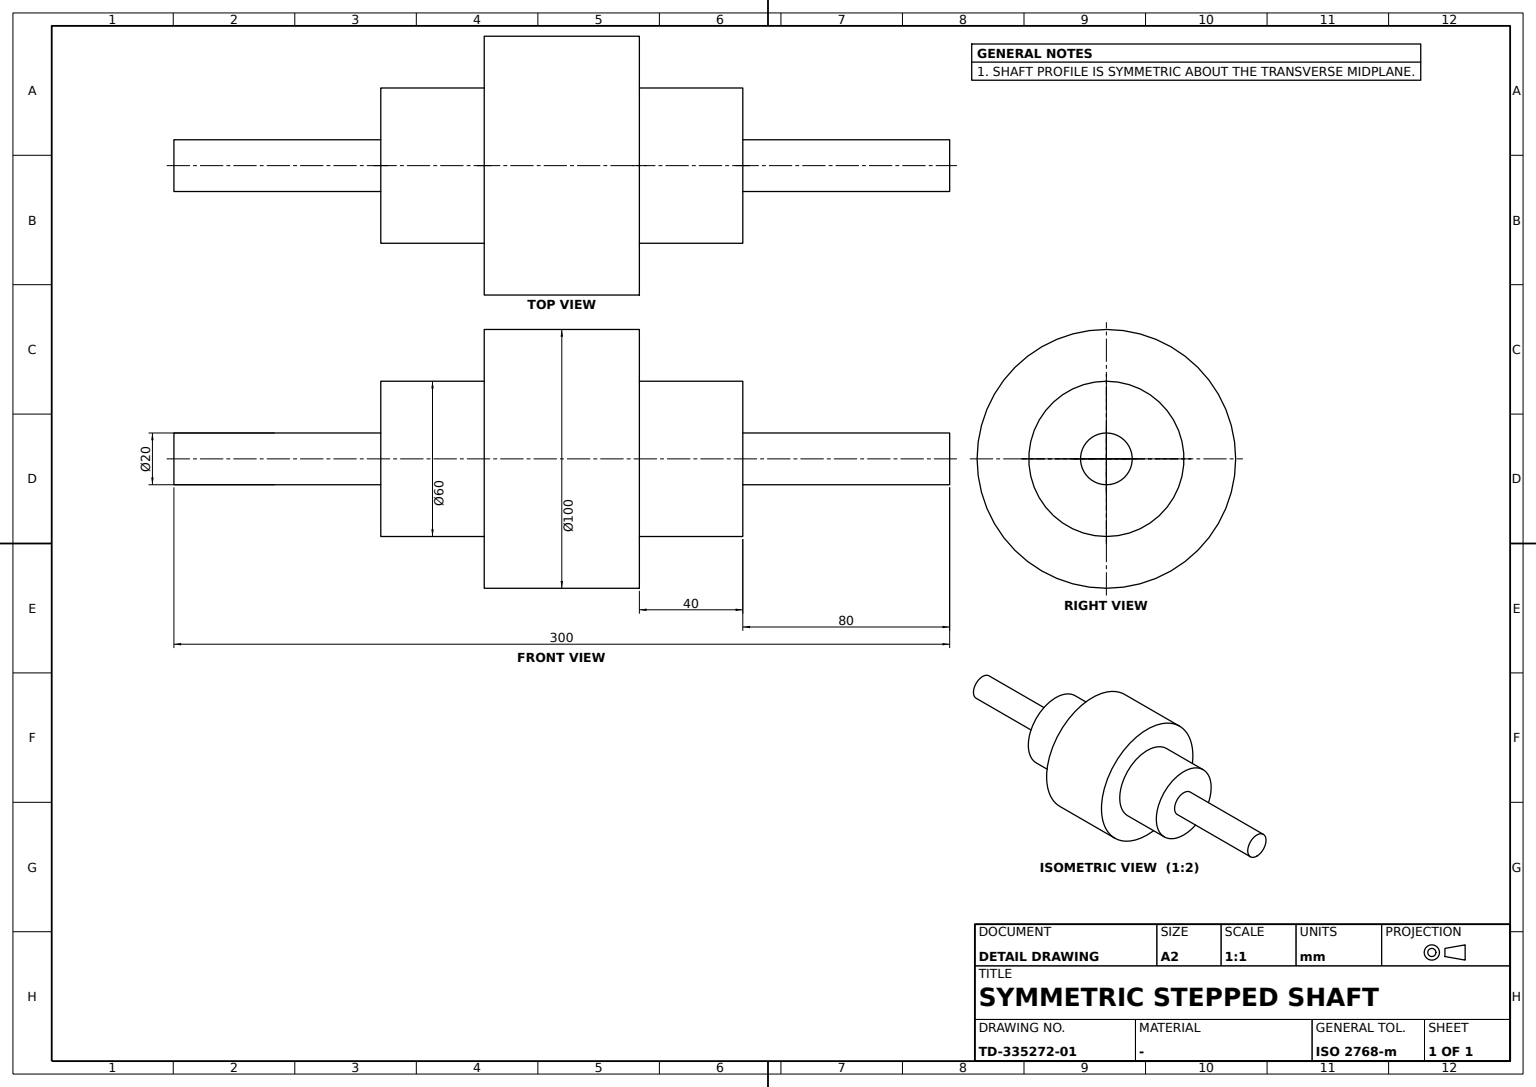
ISO-10303-21;
HEADER;
FILE_DESCRIPTION((''),'2;1');
FILE_NAME('','',(''),(''),'','','');
FILE_SCHEMA(('AUTOMOTIVE_DESIGN'));
ENDSEC;
DATA;
#1=APPLICATION_CONTEXT('');
#2=PRODUCT_CONTEXT('',#1,'mechanical');
#3=PRODUCT('','','',(#2));
#4=PRODUCT_DEFINITION_FORMATION('','',#3);
#5=PRODUCT_DEFINITION_CONTEXT('',#1,'design');
#6=PRODUCT_DEFINITION('','',#4,#5);
#7=PRODUCT_DEFINITION_SHAPE('','',#6);
#8=(LENGTH_UNIT()NAMED_UNIT(*)SI_UNIT(.MILLI.,.METRE.));
#9=(NAMED_UNIT(*)PLANE_ANGLE_UNIT()SI_UNIT($,.RADIAN.));
#10=(NAMED_UNIT(*)SI_UNIT($,.STERADIAN.)SOLID_ANGLE_UNIT());
#11=UNCERTAINTY_MEASURE_WITH_UNIT(LENGTH_MEASURE(0.005),#8,'distance_accuracy_value','');
#12=(GEOMETRIC_REPRESENTATION_CONTEXT(3)GLOBAL_UNCERTAINTY_ASSIGNED_CONTEXT((#11))GLOBAL_UNIT_ASSIGNED_CONTEXT((#8,#9,#10))REPRESENTATION_CONTEXT('',''));
#13=CARTESIAN_POINT('',(0.,-80.,-30.));
#14=VERTEX_POINT('',#13);
#15=CARTESIAN_POINT('',(0.,-80.,0.));
#16=DIRECTION('',(0.,-1.,0.));
#17=DIRECTION('',(0.,0.,-1.));
#18=AXIS2_PLACEMENT_3D('',#15,#16,#17);
#19=CIRCLE('',#18,30.);
#20=EDGE_CURVE('',#14,#14,#19,.T.);
#21=ORIENTED_EDGE('',*,*,#20,.T.);
#22=EDGE_LOOP('',(#21));
#23=FACE_BOUND('',#22,.T.);
#24=CARTESIAN_POINT('',(0.,-120.,-30.));
#25=VERTEX_POINT('',#24);
#26=CARTESIAN_POINT('',(0.,-120.,0.));
#27=AXIS2_PLACEMENT_3D('',#26,#16,#17);
#28=CIRCLE('',#27,30.);
#29=EDGE_CURVE('',#25,#25,#28,.T.);
#30=ORIENTED_EDGE('',*,*,#29,.F.);
#31=EDGE_LOOP('',(#30));
#32=FACE_BOUND('',#31,.T.);
#33=CARTESIAN_POINT('',(0.,-150.,0.));
#34=DIRECTION('',(1.,0.,0.));
#35=AXIS2_PLACEMENT_3D('',#33,#16,#34);
#36=CYLINDRICAL_SURFACE('',#35,30.);
#37=ADVANCED_FACE('',(#23,#32),#36,.T.);
#38=CARTESIAN_POINT('',(0.,-220.,-10.));
#39=VERTEX_POINT('',#38);
#40=CARTESIAN_POINT('',(0.,-220.,0.));
#41=AXIS2_PLACEMENT_3D('',#40,#16,#17);
#42=CIRCLE('',#41,10.);
#43=EDGE_CURVE('',#39,#39,#42,.T.);
#44=ORIENTED_EDGE('',*,*,#43,.T.);
#45=EDGE_LOOP('',(#44));
#46=FACE_BOUND('',#45,.T.);
#47=CARTESIAN_POINT('',(0.,-300.,-10.));
#48=VERTEX_POINT('',#47);
#49=CARTESIAN_POINT('',(0.,-300.,0.));
#50=AXIS2_PLACEMENT_3D('',#49,#16,#17);
#51=CIRCLE('',#50,10.);
#52=EDGE_CURVE('',#48,#48,#51,.T.);
#53=ORIENTED_EDGE('',*,*,#52,.F.);
#54=EDGE_LOOP('',(#53));
#55=FACE_BOUND('',#54,.T.);
#56=CYLINDRICAL_SURFACE('',#35,10.);
#57=ADVANCED_FACE('',(#46,#55),#56,.T.);
#58=CARTESIAN_POINT('',(0.,0.,-10.));
#59=VERTEX_POINT('',#58);
#60=CARTESIAN_POINT('',(0.,0.,0.));
#61=AXIS2_PLACEMENT_3D('',#60,#16,#17);
#62=CIRCLE('',#61,10.);
#63=EDGE_CURVE('',#59,#59,#62,.T.);
#64=ORIENTED_EDGE('',*,*,#63,.F.);
#65=EDGE_LOOP('',(#64));
#66=FACE_BOUND('',#65,.T.);
#67=AXIS2_PLACEMENT_3D('',#60,#16,#34);
#68=PLANE('',#67);
#69=ADVANCED_FACE('',(#66),#68,.F.);
#70=CARTESIAN_POINT('',(0.,-120.,-50.));
#71=VERTEX_POINT('',#70);
#72=CIRCLE('',#27,50.);
#73=EDGE_CURVE('',#71,#71,#72,.T.);
#74=ORIENTED_EDGE('',*,*,#73,.F.);
#75=EDGE_LOOP('',(#74));
#76=FACE_BOUND('',#75,.T.);
#77=ORIENTED_EDGE('',*,*,#29,.T.);
#78=EDGE_LOOP('',(#77));
#79=FACE_BOUND('',#78,.T.);
#80=CARTESIAN_POINT('',(0.,-120.,30.));
#81=AXIS2_PLACEMENT_3D('',#80,#16,#34);
#82=PLANE('',#81);
#83=ADVANCED_FACE('',(#76,#79),#82,.F.);
#84=ORIENTED_EDGE('',*,*,#52,.T.);
#85=EDGE_LOOP('',(#84));
#86=FACE_BOUND('',#85,.T.);
#87=CARTESIAN_POINT('',(0.,-300.,10.));
#88=AXIS2_PLACEMENT_3D('',#87,#16,#34);
#89=PLANE('',#88);
#90=ADVANCED_FACE('',(#86),#89,.T.);
#91=CARTESIAN_POINT('',(0.,-80.,-10.));
#92=VERTEX_POINT('',#91);
#93=CIRCLE('',#18,10.);
#94=EDGE_CURVE('',#92,#92,#93,.T.);
#95=ORIENTED_EDGE('',*,*,#94,.F.);
#96=EDGE_LOOP('',(#95));
#97=FACE_BOUND('',#96,.T.);
#98=ORIENTED_EDGE('',*,*,#63,.T.);
#99=EDGE_LOOP('',(#98));
#100=FACE_BOUND('',#99,.T.);
#101=ADVANCED_FACE('',(#97,#100),#56,.T.);
#102=CARTESIAN_POINT('',(0.,-180.,-50.));
#103=VERTEX_POINT('',#102);
#104=CARTESIAN_POINT('',(0.,-180.,0.));
#105=AXIS2_PLACEMENT_3D('',#104,#16,#17);
#106=CIRCLE('',#105,50.);
#107=EDGE_CURVE('',#103,#103,#106,.T.);
#108=ORIENTED_EDGE('',*,*,#107,.T.);
#109=EDGE_LOOP('',(#108));
#110=FACE_BOUND('',#109,.T.);
#111=CARTESIAN_POINT('',(0.,-180.,-30.));
#112=VERTEX_POINT('',#111);
#113=CIRCLE('',#105,30.);
#114=EDGE_CURVE('',#112,#112,#113,.T.);
#115=ORIENTED_EDGE('',*,*,#114,.F.);
#116=EDGE_LOOP('',(#115));
#117=FACE_BOUND('',#116,.T.);
#118=CARTESIAN_POINT('',(0.,-180.,50.));
#119=AXIS2_PLACEMENT_3D('',#118,#16,#34);
#120=PLANE('',#119);
#121=ADVANCED_FACE('',(#110,#117),#120,.T.);
#122=ORIENTED_EDGE('',*,*,#43,.F.);
#123=EDGE_LOOP('',(#122));
#124=FACE_BOUND('',#123,.T.);
#125=CARTESIAN_POINT('',(0.,-220.,-30.));
#126=VERTEX_POINT('',#125);
#127=CIRCLE('',#41,30.);
#128=EDGE_CURVE('',#126,#126,#127,.T.);
#129=ORIENTED_EDGE('',*,*,#128,.T.);
#130=EDGE_LOOP('',(#129));
#131=FACE_BOUND('',#130,.T.);
#132=CARTESIAN_POINT('',(0.,-220.,30.));
#133=AXIS2_PLACEMENT_3D('',#132,#16,#34);
#134=PLANE('',#133);
#135=ADVANCED_FACE('',(#124,#131),#134,.T.);
#136=ORIENTED_EDGE('',*,*,#73,.T.);
#137=EDGE_LOOP('',(#136));
#138=FACE_BOUND('',#137,.T.);
#139=ORIENTED_EDGE('',*,*,#107,.F.);
#140=EDGE_LOOP('',(#139));
#141=FACE_BOUND('',#140,.T.);
#142=CYLINDRICAL_SURFACE('',#35,50.);
#143=ADVANCED_FACE('',(#138,#141),#142,.T.);
#144=ORIENTED_EDGE('',*,*,#20,.F.);
#145=EDGE_LOOP('',(#144));
#146=FACE_BOUND('',#145,.T.);
#147=ORIENTED_EDGE('',*,*,#94,.T.);
#148=EDGE_LOOP('',(#147));
#149=FACE_BOUND('',#148,.T.);
#150=CARTESIAN_POINT('',(0.,-80.,10.));
#151=AXIS2_PLACEMENT_3D('',#150,#16,#34);
#152=PLANE('',#151);
#153=ADVANCED_FACE('',(#146,#149),#152,.F.);
#154=ORIENTED_EDGE('',*,*,#128,.F.);
#155=EDGE_LOOP('',(#154));
#156=FACE_BOUND('',#155,.T.);
#157=ORIENTED_EDGE('',*,*,#114,.T.);
#158=EDGE_LOOP('',(#157));
#159=FACE_BOUND('',#158,.T.);
#160=ADVANCED_FACE('',(#156,#159),#36,.T.);
#161=CLOSED_SHELL('',(#37,#57,#69,#83,#90,#101,#121,#135,#143,#153,#160));
#162=MANIFOLD_SOLID_BREP('',#161);
#163=ADVANCED_BREP_SHAPE_REPRESENTATION('',(#162),#12);
#164=SHAPE_DEFINITION_REPRESENTATION(#7,#163);
ENDSEC;
END-ISO-10303-21;
